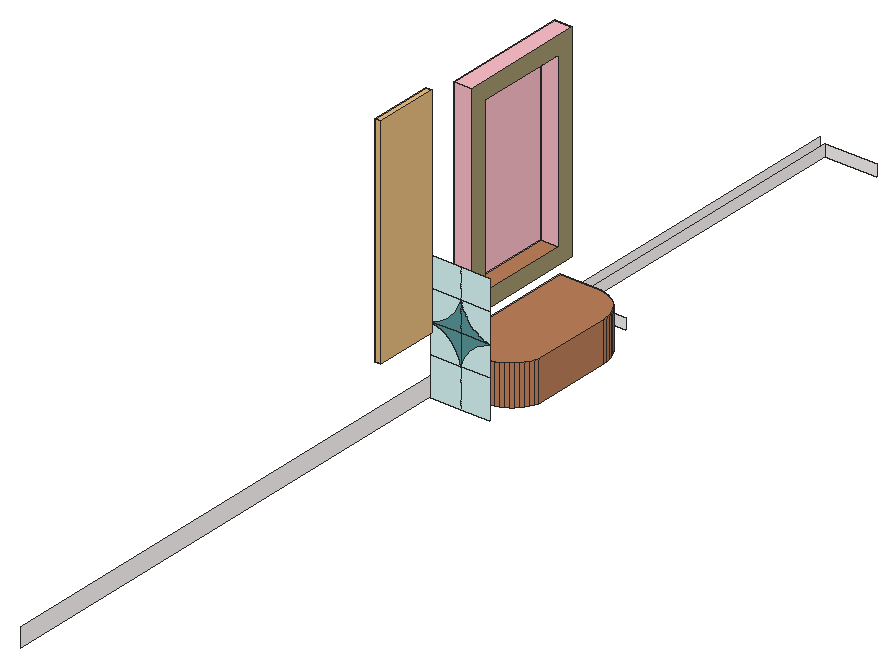
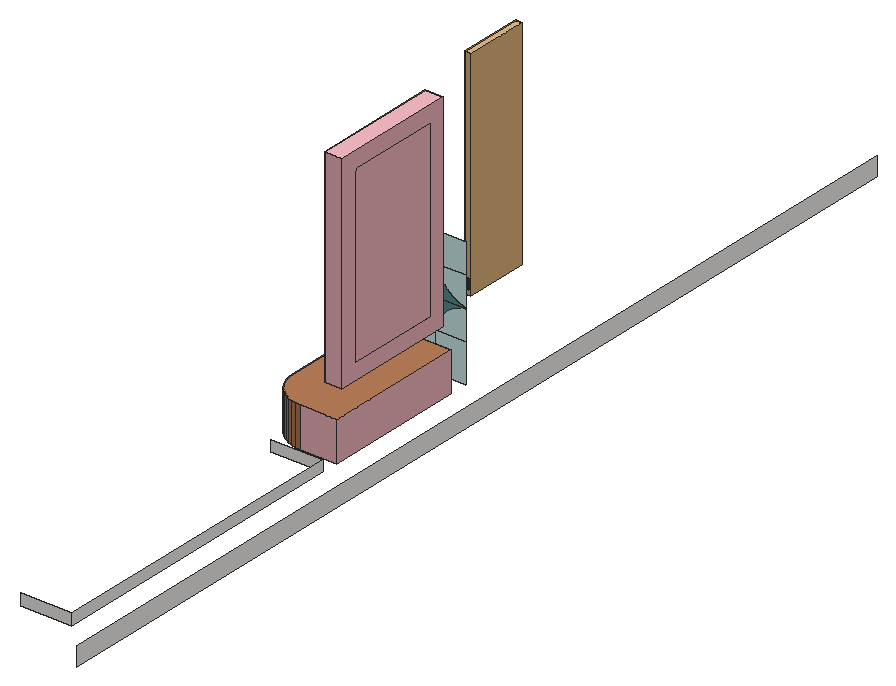
# SketchUp Ruby script. Lengths in inches.
U = 1.inch
M = Sketchup.active_model
def pt(a) = Geom::Point3d.new(a.map { |v| v * U })
def face(e, loops, mat)
  f = e.add_face(loops[0].map { |a| pt(a) })
  loops[1..].each { |l| e.add_face(l.map { |a| pt(a) }).erase! }
  f.material = f.back_material = mat if mat
  f
end
# faces: each face lists its corners as indices into pts; further lists are holes
def faces(e, pts, list, mat = nil) = list.each { |f| face(e, (f[0].is_a?(Array) ? f : [f]).map { |l| l.map { |i| pts[i] } }, mat) }
# xy, xz, yz: faces in a plane at the given z, y or x. An outline is a flat list of corners, or four numbers for a rectangle; further outlines are holes
def ring(l) = l.size == 4 ? [[l[0], l[1]], [l[2], l[1]], [l[2], l[3]], [l[0], l[3]]] : l.each_slice(2).to_a
def flat(e, list, mat, &to3) = list.each { |f| face(e, (f[0].is_a?(Array) ? f : [f]).map { |l| ring(l).map { |u, v| to3.(u, v) } }, mat) }
def xy(e, z, list, mat = nil) = flat(e, list, mat) { |x, y| [x, y, z] }
def xz(e, y, list, mat = nil) = flat(e, list, mat) { |x, z| [x, y, z] }
def yz(e, x, list, mat = nil) = flat(e, list, mat) { |y, z| [x, y, z] }
def lines(e, pts, list) = list.each { |a, b| e.add_line(pt(pts[a]), pt(pts[b])) }
# prism: a flat outline (further loops are holes) pulled along v
def prism(e, loops, v, mat = nil)
  f = face(e, loops, mat); d = Geom::Vector3d.new(v.map { |x| x * U })
  f.pushpull(f.normal.samedirection?(d) ? d.length : -d.length)
end
def box(e, o, s, mat = nil) = prism(e, [[o, [o[0] + s[0], o[1], o[2]], [o[0] + s[0], o[1] + s[1], o[2]], [o[0], o[1] + s[1], o[2]]]], [0, 0, s[2]], mat)
def at(x, y, z, deg = 0) = Geom::Transformation.translation(pt([x, y, z])) * Geom::Transformation.rotation(ORIGIN, Z_AXIS, deg.degrees)
def axes(o, x, y, z) = Geom::Transformation.new([*x, 0, *y, 0, *z, 0, *pt(o).to_a, 1])
def part(name) = M.definitions.add(name)
# library, detail: a bought-in or finely detailed component or shape, given as its bounding box
def library(name, o, s) = part(name).tap { |d| box(d.entities, o, s) }
def detail(e, o, s) = box(e.add_group.entities, o, s)
def put(e, d, t, mat = nil) = e.add_instance(d, t).tap { |i| i.material = mat if mat }
def group(e, t, mat = nil) = e.add_group.tap { |g| g.transformation = t; g.material = mat if mat }.entities
root = M.entities
M.materials.add("3D66_SU_1584934530570_001").color = [198, 166, 120]
M.materials.add("3D66_SU_1584934530605_002").color = [112, 126, 151]
M.materials.add("[0006_Pink]").color = [255, 192, 203]
M.materials.add("[0010_Snow]").color = [255, 250, 250]
M.materials.add("[0081_CadetBlue]").color = [95, 158, 160]
M.materials.add("[0090_LightCyan]").color = [224, 255, 255]
M.materials.add("[Wood Lumber ButtJoined]").color = [164, 152, 112]
M.materials.add("[Wood Veneer 02]").color = [190, 128, 91]
c1 = part("\#56")
xy(c1.entities,-100.5,[[4101.68,3813.38,4458.05,3883.7]],"3D66_SU_1584934530570_001")
xy(c1.entities,-87.5,[[4103.64,3815.34,4456.09,3881.74]],"3D66_SU_1584934530570_001")
xz(c1.entities,3813.38,[[4101.68,-100.5,4458.05,-90.5]],"3D66_SU_1584934530570_001")
xz(c1.entities,3883.7,[[4101.68,-100.5,4458.05,-90.5]],"3D66_SU_1584934530570_001")
yz(c1.entities,4101.68,[[3813.38,-100.5,3883.7,-90.5]],"3D66_SU_1584934530570_001")
yz(c1.entities,4458.05,[[3813.38,-100.5,3883.7,-90.5]],"3D66_SU_1584934530570_001")
p = [[4101.68,3883.7,-90.5],[4101.68,3813.38,-90.5],[4103.64,3815.34,-87.5],[4103.64,3881.74,-87.5],[4458.05,3813.38,-90.5],[4456.09,3815.34,-87.5],
  [4458.05,3883.7,-90.5],[4456.09,3881.74,-87.5]]
faces(c1.entities,p,[[0,1,2,3],[1,4,5,2],[4,6,7,5],[6,0,3,7]],"3D66_SU_1584934530570_001")
c2 = library("\#55",[4102.66,3775.67,-115.5],[369.45,1517.42,40])
xy(root,0,[[118.5625,341.67,118.5625,398.98,133.16,398.98,135.02,398.86,136.85,398.49,138.62,397.89,140.3,397.07,141.85,396.03,143.25,394.8,144.49,393.39,145.52,391.84,146.35,390.16,146.95,388.39,147.32,386.5625,147.4375,384.7,147.4375,352.32,146.88,350.8125,146.18,349.38,145.32,348.03,144.33,346.78,143.21,345.63,141.97,344.62,140.63,343.74,139.21,343,137.72,342.42,136.18,342.01,134.6,341.75,133,341.67]],"[0006_Pink]")
xy(root,16,[[118.5625,341.67,133,341.67,134.6,341.75,136.18,342.01,137.72,342.42,139.21,343,140.63,343.74,141.97,344.62,143.21,345.63,144.33,346.78,145.32,348.03,146.18,349.38,146.88,350.8125,147.4375,352.32,147.4375,384.7,147.32,386.5625,146.95,388.39,146.35,390.16,145.52,391.84,144.49,393.39,143.25,394.8,141.85,396.03,140.3,397.07,138.62,397.89,136.85,398.49,135.02,398.86,133.16,398.98,118.5625,398.98]],"[Wood Veneer 02]")
xy(root,25.77,[[118.5625,345.56,125.6875,396.18]],"[0006_Pink]")
xy(root,32.6,[[118.5625,352.39,125.6875,389.35]],"[Wood Veneer 02]")
xy(root,101.87,[[118.5625,352.39,125.6875,389.35]],"[0006_Pink]")
xy(root,108.7,[[118.5625,345.56,125.6875,396.18]],"[0006_Pink]")
xz(root,333.9375,[[130.5625,15.41,130.5625,27.41,118.5625,27.41,120.05,27.11,121.49,26.65,122.88,26.05,124.2,25.3,125.42,24.41,126.55,23.4,127.5625,22.27,128.45,21.04,129.2,19.73,129.81,18.34,130.26,16.89],[130.5625,15.41,131.05,16.8,131.64,18.14,132.35,19.4375,133.16,20.67,134.0625,21.83,135.06,22.91,136.14,23.91,137.3,24.8125,138.53,25.62,139.83,26.33,141.17,26.92,142.5625,27.41,130.5625,27.41],[118.5625,27.41,130.5625,27.41,130.5625,39.41,130.16,37.97,129.63,36.58,128.97,35.25,128.1875,33.98,127.29,32.79,126.29,31.68,125.18,30.68,123.99,29.78,122.73,29,121.39,28.34,120,27.81],[130.5625,27.41,142.5625,27.41,141.14,27.83,139.75,28.37,138.43,29.04,137.17,29.83,135.98,30.73,134.88,31.73,133.88,32.83,132.98,34.01,132.2,35.27,131.53,36.6,130.98,37.98,130.5625,39.41]],"[0081_CadetBlue]")
xz(root,333.9375,[[118.5625,0,130.5625,15.41],[130.5625,0,142.5625,15.41],[118.5625,15.41,130.5625,15.41,130.26,16.89,129.81,18.34,129.2,19.73,128.45,21.04,127.5625,22.27,126.55,23.4,125.42,24.41,124.2,25.3,122.88,26.05,121.49,26.65,120.05,27.11,118.5625,27.41],[130.5625,15.41,142.5625,15.41,142.5625,27.41,141.17,26.92,139.83,26.33,138.53,25.62,137.3,24.8125,136.14,23.91,135.06,22.91,134.0625,21.83,133.16,20.67,132.35,19.4375,131.64,18.14,131.05,16.8],[118.5625,27.41,120,27.81,121.39,28.34,122.73,29,123.99,29.78,125.18,30.68,126.29,31.68,127.29,32.79,128.1875,33.98,128.97,35.25,129.63,36.58,130.16,37.97,130.5625,39.41,118.5625,39.41],
  [142.5625,27.41,142.5625,39.41,130.5625,39.41,130.98,37.98,131.53,36.6,132.2,35.27,132.98,34.01,133.88,32.83,134.88,31.73,135.98,30.73,137.17,29.83,138.43,29.04,139.75,28.37,141.14,27.83],[118.5625,39.41,130.5625,51.41],[130.5625,39.41,142.5625,51.41]],"[0090_LightCyan]")
xz(root,341.67,[[118.5625,0,133,16]],"[0006_Pink]")
xz(root,345.56,[[118.5625,25.77,125.6875,108.7]],"[0006_Pink]")
xz(root,352.39,[[118.5625,32.6,125.6875,101.87]],"[0006_Pink]")
xz(root,389.35,[[118.5625,32.6,125.6875,101.87]],"[0006_Pink]")
xz(root,396.18,[[118.5625,25.77,125.6875,108.7]],"[0006_Pink]")
xz(root,398.98,[[118.5625,0,133.16,16]],"[0006_Pink]")
xz(root,405.9375,[[118.5625,0,139.41,4.5]],"[0010_Snow]")
xz(root,531.9375,[[118.5625,0,139.41,4.5]],"[0010_Snow]")
yz(root,109.5625,[[138.9375,-7.5625,540.9375,0]],"[0010_Snow]")
yz(root,118.5625,[[341.67,0,398.98,16],[[345.56,25.77,396.18,108.7],[352.39,32.6,389.35,101.87]],[352.39,32.6,389.35,101.87]],"[0006_Pink]")
yz(root,118.5625,[[405.9375,0,531.9375,4.5]],"[0010_Snow]")
yz(root,122.5,[[309.36,41.39,306.33,48.97,309.47,41.43],[309.47,41.43,306.33,48.97,309.59,41.47],[309.59,41.47,306.56,49.03,309.84,41.54],[309.84,41.54,306.67,49.07,310.1,41.6],[310.1,41.6,306.88,49.16,310.375,41.64],
  [310.375,41.64,306.99,49.22,310.95,41.72],[310.95,41.72,306.99,49.22,307.2,49.33],[310.95,41.72,307.2,49.33,307.41,49.46],[310.95,41.72,307.41,49.46,311.54,41.77],[311.54,41.77,307.41,49.46,307.61,49.6],
  [311.54,41.77,307.61,49.6,312.72,41.83],[312.72,41.83,307.61,49.6,307.81,49.75],[312.72,41.83,307.81,49.75,308.19,50.06],[312.72,41.83,308.19,50.06,313.27,41.87],[313.27,41.87,308.19,50.06,308.92,50.67],
  [313.27,41.87,308.92,50.67,313.78,41.92],[313.78,41.92,308.92,50.67,314.26,41.97],[314.26,41.97,308.92,50.67,309.27,50.94],[314.26,41.97,309.27,50.94,309.44,51.06],[314.26,41.97,309.44,51.06,309.53,51.11],
  [314.26,41.97,309.53,51.11,309.61,51.16],[314.26,41.97,309.61,51.16,309.93,51.32],[314.26,41.97,309.93,51.32,310.23,51.46],[314.26,41.97,310.23,51.46,310.51,51.58],[314.26,41.97,310.51,51.58,310.79,51.68],
  [314.26,41.97,310.79,51.68,311.06,51.76],[314.26,41.97,311.06,51.76,311.34,51.83],[314.26,41.97,311.34,51.83,311.63,51.89],[314.26,41.97,311.63,51.89,311.94,51.9375],[314.26,41.97,311.94,51.9375,312.11,51.96],
  [314.26,41.97,312.11,51.96,312.29,51.98],[314.26,41.97,312.29,51.98,312.65,52],[314.26,41.97,312.65,52,313.02,52],[314.26,41.97,313.02,52,313.4,52],[314.26,41.97,313.4,52,314.84,51.92],
  [314.26,41.97,314.84,51.92,314.73,42],[314.73,42,314.84,51.92,315,51.91],[314.73,42,315,51.91,315.15,51.89],[314.73,42,315.15,51.89,315.45,51.84],[314.73,42,315.45,51.84,316.01,51.72],
  [314.73,42,316.01,51.72,315.6,42.06],[315.6,42.06,316.01,51.72,316.27,51.67],[315.6,42.06,316.27,51.67,316.01,42.1],[316.01,42.1,316.27,51.67,316.4,51.64],[316.01,42.1,316.4,51.64,316.21,42.12],
  [316.21,42.12,316.4,51.64,316.4,42.15],[316.4,42.15,316.4,51.64,316.59,42.19],[316.59,42.19,316.4,51.64,316.77,42.24],[316.77,42.24,316.4,51.64,316.86,42.26],[316.86,42.26,316.4,51.64,316.94,42.29],
  [316.94,42.29,316.4,51.64,317.03,42.32],[317.03,42.32,316.4,51.64,317.11,42.36],[317.11,42.36,316.4,51.64,317.27,42.43],[317.27,42.43,316.4,51.64,317.41,42.51],[317.41,42.51,316.4,51.64,317.55,42.6],
  [317.55,42.6,316.4,51.64,317.69,42.69],[317.69,42.69,316.4,51.64,317.81,42.79],[317.81,42.79,316.4,51.64,317.93,42.9],[317.93,42.9,316.4,51.64,318.04,43.01],[318.04,43.01,316.4,51.64,318.15,43.12],
  [318.15,43.12,316.4,51.64,319,44.16],[319,44.16,316.4,51.64,319.43,44.73],[319.43,44.73,316.4,51.64,319.84,45.34],[319.84,45.34,316.4,51.64,320.78,46.84]],"3D66_SU_1584934530605_002")
yz(root,123.07,[[309.36,41.39,309.47,41.43,306.33,48.97],[309.47,41.43,309.59,41.47,306.33,48.97],[309.59,41.47,309.84,41.54,306.56,49.03],[309.84,41.54,310.1,41.6,306.67,49.07],[310.1,41.6,310.375,41.64,306.88,49.16],
  [310.375,41.64,310.95,41.72,306.99,49.22],[310.95,41.72,307.2,49.33,306.99,49.22],[310.95,41.72,307.41,49.46,307.2,49.33],[310.95,41.72,311.54,41.77,307.41,49.46],[311.54,41.77,307.61,49.6,307.41,49.46],
  [311.54,41.77,312.72,41.83,307.61,49.6],[312.72,41.83,307.81,49.75,307.61,49.6],[312.72,41.83,308.19,50.06,307.81,49.75],[312.72,41.83,313.27,41.87,308.19,50.06],[313.27,41.87,308.92,50.67,308.19,50.06],
  [313.27,41.87,313.78,41.92,308.92,50.67],[313.78,41.92,314.26,41.97,308.92,50.67],[314.26,41.97,309.27,50.94,308.92,50.67],[314.26,41.97,309.44,51.06,309.27,50.94],[314.26,41.97,309.53,51.11,309.44,51.06],
  [314.26,41.97,309.61,51.16,309.53,51.11],[314.26,41.97,309.93,51.32,309.61,51.16],[314.26,41.97,310.23,51.46,309.93,51.32],[314.26,41.97,310.51,51.58,310.23,51.46],[314.26,41.97,310.79,51.68,310.51,51.58],
  [314.26,41.97,311.06,51.76,310.79,51.68],[314.26,41.97,311.34,51.83,311.06,51.76],[314.26,41.97,311.63,51.89,311.34,51.83],[314.26,41.97,311.94,51.9375,311.63,51.89],[314.26,41.97,312.11,51.96,311.94,51.9375],
  [314.26,41.97,312.29,51.98,312.11,51.96],[314.26,41.97,312.65,52,312.29,51.98],[314.26,41.97,313.02,52,312.65,52],[314.26,41.97,313.4,52,313.02,52],[314.26,41.97,314.84,51.92,313.4,52],
  [314.26,41.97,314.73,42,314.84,51.92],[314.73,42,315,51.91,314.84,51.92],[314.73,42,315.15,51.89,315,51.91],[314.73,42,315.45,51.84,315.15,51.89],[314.73,42,315.6,42.06,316.01,51.72],
  [314.73,42,316.01,51.72,315.45,51.84],[315.6,42.06,316.01,42.1,316.27,51.67],[315.6,42.06,316.27,51.67,316.01,51.72],[316.01,42.1,316.21,42.12,316.4,51.64],[316.01,42.1,316.4,51.64,316.27,51.67],
  [316.21,42.12,316.4,42.15,316.4,51.64],[316.4,42.15,316.59,42.19,316.4,51.64],[316.59,42.19,316.77,42.24,316.4,51.64],[316.77,42.24,316.86,42.26,316.4,51.64],[316.86,42.26,316.94,42.29,316.4,51.64],
  [316.94,42.29,317.03,42.32,316.4,51.64],[317.03,42.32,317.11,42.36,316.4,51.64],[317.11,42.36,317.27,42.43,316.4,51.64],[317.27,42.43,317.41,42.51,316.4,51.64],[317.41,42.51,317.55,42.6,316.4,51.64],
  [317.55,42.6,317.69,42.69,316.4,51.64],[317.69,42.69,317.81,42.79,316.4,51.64],[317.81,42.79,317.93,42.9,316.4,51.64],[317.93,42.9,318.04,43.01,316.4,51.64],[318.04,43.01,318.15,43.12,316.4,51.64],
  [318.15,43.12,319,44.16,316.4,51.64],[319,44.16,319.43,44.73,316.4,51.64],[319.43,44.73,319.84,45.34,316.4,51.64],[319.84,45.34,320.78,46.84,316.4,51.64]],"3D66_SU_1584934530605_002")
yz(root,125.6875,[[[345.56,25.77,396.18,108.7],[352.39,32.6,389.35,101.87]]],"[Wood Lumber ButtJoined]")
yz(root,147.4375,[[352.32,0,384.7,16]],"[Wood Veneer 02]")
p = [[134.6,341.75,16],[133,341.67,16],[133,341.67,0],[134.6,341.75,0],[136.18,342.01,16],[136.18,342.01,0],
  [137.72,342.42,16],[137.72,342.42,0],[139.21,343,16],[139.21,343,0],[140.63,343.74,16],[140.63,343.74,0],
  [141.97,344.62,16],[141.97,344.62,0],[143.21,345.63,16],[143.21,345.63,0],[144.33,346.78,16],[144.33,346.78,0],
  [145.32,348.03,16],[145.32,348.03,0],[146.18,349.38,16],[146.18,349.38,0],[146.88,350.8125,16],[146.88,350.8125,0],
  [147.4375,352.32,16],[147.4375,352.32,0],[147.32,386.5625,16],[147.4375,384.7,16],[147.4375,384.7,0],[147.32,386.5625,0],
  [146.95,388.39,16],[146.95,388.39,0],[146.35,390.16,16],[146.35,390.16,0],[145.52,391.84,16],[145.52,391.84,0],
  [144.49,393.39,16],[144.49,393.39,0],[143.25,394.8,16],[143.25,394.8,0],[141.85,396.03,16],[141.85,396.03,0],
  [140.3,397.07,16],[140.3,397.07,0],[138.62,397.89,16],[138.62,397.89,0],[136.85,398.49,16],[136.85,398.49,0],
  [135.02,398.86,16],[135.02,398.86,0],[133.16,398.98,16],[133.16,398.98,0],[123.07,308.4,40.91],[122.5,308.4,40.91],
  [122.5,308.57,41.02],[123.07,308.57,41.02],[122.5,308.75,41.12],[123.07,308.75,41.12],[122.5,308.9375,41.21],[123.07,308.9375,41.21],
  [122.5,309.14,41.3],[123.07,309.14,41.3],[122.5,309.36,41.39],[123.07,309.36,41.39],[122.5,309.47,41.43],[123.07,309.47,41.43],
  [122.5,309.59,41.47],[123.07,309.59,41.47],[122.5,309.84,41.54],[123.07,309.84,41.54],[122.5,310.1,41.6],[123.07,310.1,41.6],
  [122.5,310.375,41.64],[123.07,310.375,41.64],[122.5,310.95,41.72],[123.07,310.95,41.72],[122.5,311.54,41.77],[123.07,311.54,41.77],
  [122.5,312.72,41.83],[123.07,312.72,41.83],[122.5,313.27,41.87],[123.07,313.27,41.87],[122.5,313.78,41.92],[123.07,313.78,41.92],
  [122.5,314.26,41.97],[123.07,314.26,41.97],[122.5,314.73,42],[123.07,314.73,42],[122.5,315.6,42.06],[123.07,315.6,42.06],
  [122.5,316.01,42.1],[123.07,316.01,42.1],[122.5,316.21,42.12],[123.07,316.21,42.12],[122.5,316.4,42.15],[123.07,316.4,42.15],
  [122.5,316.59,42.19],[123.07,316.59,42.19],[122.5,316.77,42.24],[123.07,316.77,42.24],[122.5,316.86,42.26],[123.07,316.86,42.26],
  [122.5,316.94,42.29],[123.07,316.94,42.29],[122.5,317.03,42.32],[123.07,317.03,42.32],[122.5,317.11,42.36],[123.07,317.11,42.36],
  [122.5,317.27,42.43],[123.07,317.27,42.43],[122.5,317.41,42.51],[123.07,317.41,42.51],[122.5,317.55,42.6],[123.07,317.55,42.6],
  [122.5,317.69,42.69],[123.07,317.69,42.69],[122.5,317.81,42.79],[123.07,317.81,42.79],[122.5,317.93,42.9],[123.07,317.93,42.9],
  [122.5,318.04,43.01],[123.07,318.04,43.01],[122.5,318.15,43.12],[123.07,318.15,43.12],[122.5,319,44.16],[123.07,319,44.16],
  [122.5,319.43,44.73],[123.07,319.43,44.73],[122.5,319.84,45.34],[123.07,319.84,45.34],[122.5,320.78,46.84],[123.07,320.78,46.84]]
faces(root,p,[[0,1,2,3],[4,0,3,5],[6,4,5,7],[8,6,7,9],[10,8,9,11],[12,10,11,13],[14,12,13,15],[16,14,15,17],
  [18,16,17,19],[20,18,19,21],[22,20,21,23],[24,22,23,25],[26,27,28,29],[30,26,29,31],[32,30,31,33],[34,32,33,35],
  [36,34,35,37],[38,36,37,39],[40,38,39,41],[42,40,41,43],[44,42,43,45],[46,44,45,47],[48,46,47,49],[50,48,49,51]],"[Wood Veneer 02]")
faces(root,p,[[52,53,54,55],[55,54,56,57],[57,56,58,59],[59,58,60,61],[61,60,62,63],[63,62,64,65],[65,64,66,67],[67,66,68,69],
  [69,68,70,71],[71,70,72,73],[73,72,74,75],[75,74,76,77],[77,76,78,79],[79,78,80,81],[81,80,82,83],[83,82,84,85],
  [85,84,86,87],[87,86,88,89],[89,88,90,91],[91,90,92,93],[93,92,94,95],[95,94,96,97],[97,96,98,99],[99,98,100,101],
  [101,100,102,103],[103,102,104,105],[105,104,106,107],[107,106,108,109],[109,108,110,111],[111,110,112,113],[113,112,114,115],[115,114,116,117],
  [117,116,118,119],[119,118,120,121],[121,120,122,123],[123,122,124,125],[125,124,126,127],[127,126,128,129],[129,128,130,131]],"3D66_SU_1584934530605_002")
put(root,c1,axes([117.28,611.37,-189.42],[0,-0.06912,0],[0,0,0.0576],[-0.0576,0,0]),"3D66_SU_1584934530570_001")
put(root,c2,axes([117.28,611.37,-189.42],[0,-0.06912,0],[0,0,0.0576],[-0.0576,0,0]),"3D66_SU_1584934530570_001")
